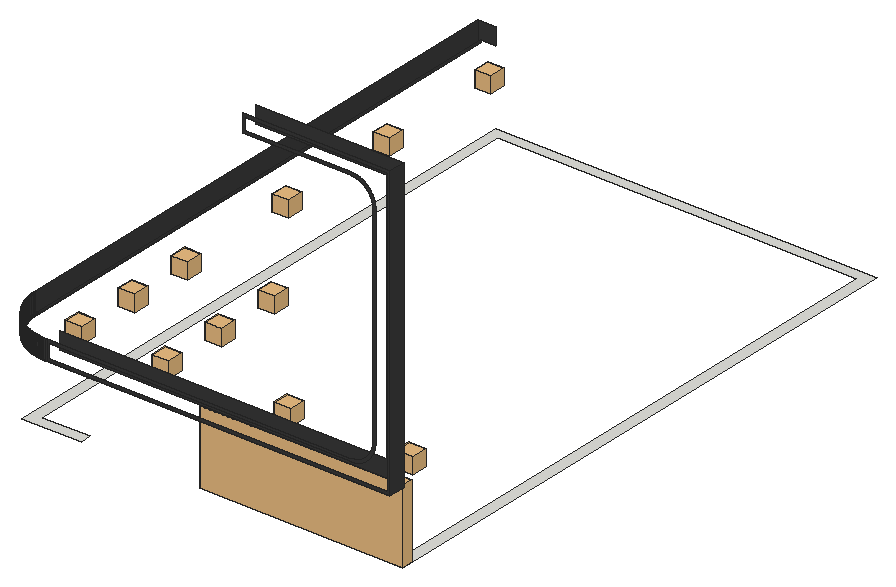
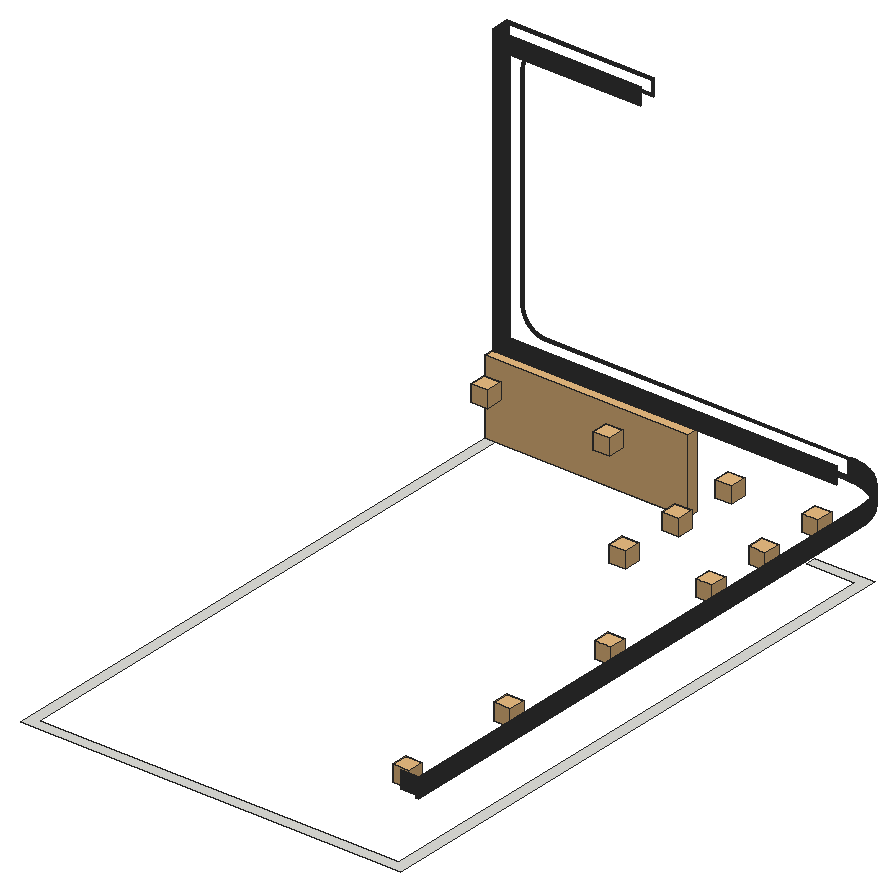
# SketchUp Ruby script. Lengths in inches.
U = 1.inch
M = Sketchup.active_model
def pt(a) = Geom::Point3d.new(a.map { |v| v * U })
def face(e, loops, mat)
  f = e.add_face(loops[0].map { |a| pt(a) })
  loops[1..].each { |l| e.add_face(l.map { |a| pt(a) }).erase! }
  f.material = f.back_material = mat if mat
  f
end
# faces: each face lists its corners as indices into pts; further lists are holes
def faces(e, pts, list, mat = nil) = list.each { |f| face(e, (f[0].is_a?(Array) ? f : [f]).map { |l| l.map { |i| pts[i] } }, mat) }
# xy, xz, yz: faces in a plane at the given z, y or x. An outline is a flat list of corners, or four numbers for a rectangle; further outlines are holes
def ring(l) = l.size == 4 ? [[l[0], l[1]], [l[2], l[1]], [l[2], l[3]], [l[0], l[3]]] : l.each_slice(2).to_a
def flat(e, list, mat, &to3) = list.each { |f| face(e, (f[0].is_a?(Array) ? f : [f]).map { |l| ring(l).map { |u, v| to3.(u, v) } }, mat) }
def xy(e, z, list, mat = nil) = flat(e, list, mat) { |x, y| [x, y, z] }
def xz(e, y, list, mat = nil) = flat(e, list, mat) { |x, z| [x, y, z] }
def yz(e, x, list, mat = nil) = flat(e, list, mat) { |y, z| [x, y, z] }
def lines(e, pts, list) = list.each { |a, b| e.add_line(pt(pts[a]), pt(pts[b])) }
# prism: a flat outline (further loops are holes) pulled along v
def prism(e, loops, v, mat = nil)
  f = face(e, loops, mat); d = Geom::Vector3d.new(v.map { |x| x * U })
  f.pushpull(f.normal.samedirection?(d) ? d.length : -d.length)
end
def box(e, o, s, mat = nil) = prism(e, [[o, [o[0] + s[0], o[1], o[2]], [o[0] + s[0], o[1] + s[1], o[2]], [o[0], o[1] + s[1], o[2]]]], [0, 0, s[2]], mat)
def at(x, y, z, deg = 0) = Geom::Transformation.translation(pt([x, y, z])) * Geom::Transformation.rotation(ORIGIN, Z_AXIS, deg.degrees)
def axes(o, x, y, z) = Geom::Transformation.new([*x, 0, *y, 0, *z, 0, *pt(o).to_a, 1])
def part(name) = M.definitions.add(name)
# library, detail: a bought-in or finely detailed component or shape, given as its bounding box
def library(name, o, s) = part(name).tap { |d| box(d.entities, o, s) }
def detail(e, o, s) = box(e.add_group.entities, o, s)
def put(e, d, t, mat = nil) = e.add_instance(d, t).tap { |i| i.material = mat if mat }
def group(e, t, mat = nil) = e.add_group.tap { |g| g.transformation = t; g.material = mat if mat }.entities
root = M.entities
M.materials.add("1496 AP 8293 CARBON COPY").color = [58, 58, 58]
c1 = library("Group\#5",[0,0,0],[165,9,60])
c2 = library("2",[-4.69,-4.69,-13.16],[13.38,13.38,13.16])
xy(root,69,[[14,84,62,84,62,93,23,93,23,555,314,555,314,93,158,93,158,84,323,84,323,564,14,564]])
xy(root,127,[[43.42,71,42.85,71.02,42.27,71.03,41.7,71.06,41.12,71.09,40.55,71.14,39.97,71.18,38.83,71.3,38.26,71.375,37.6875,71.46,37.12,71.54,35.98,71.74,35.42,71.85,34.85,71.96,34.29,72.08,33.73,72.22,33.17,72.35,32.61,72.5,32.06,72.65,31.5,72.8125,30.95,72.98,30.4,73.15,29.86,73.34,29.3125,73.52,28.77,73.72,28.23,73.92,27.7,74.13,27.16,74.35,26.63,74.57,26.1,74.8,25.58,75.04,24.54,75.54,24.02,75.8,23.51,76.0625,23.01,76.33,22.5,76.61,22,76.89,21.5,77.1875,21.01,77.48,20.52,77.79,20.04,78.1,19.55,78.42,19.08,78.74,18.14,79.4,17.67,79.74,17.21,80.09,15.86,81.17,15.42,81.54,14.56,82.3,14.13,82.69,13.71,83.08,13.3,83.48,12.48,84.3,12.08,84.71,11.69,85.13,11.3,85.56,10.54,86.42,10.17,86.86,9.09,88.21,8.74,88.67,8.4,89.14,7.74,90.08,7.42,90.55,7.1,91.04,6.79,91.52,6.48,92.01,6.1875,92.5,5.89,93,5.61,93.5,5.33,94.01,5.0625,94.51,4.8,95.02,4.54,95.54,4.04,96.58,3.8,97.1,3.57,97.63,3.35,98.16,3.13,98.7,2.92,99.23,2.72,99.77,2.52,100.3125,2.34,100.86,2.15,101.4,1.98,101.95,1.8125,102.5,1.65,103.06,1.5,103.61,1.35,104.17,1.22,104.73,1.08,105.29,0.96,105.85,0.85,106.42,0.74,106.98,0.54,108.12,0.46,108.6875,0.375,109.26,0.3,109.83,0.18,110.97,0.14,111.55,0.09,112.12,0.06,112.7,0.03,113.27,0.02,113.85,0,114.42,0,564,2,564,2,114.45,2.01,113.9,2.03,113.35,2.09,112.25,2.13,111.7,2.18,111.16,2.23,110.61,2.29,110.0625,2.36,109.52,2.43,108.97,2.7,107.35,2.92,106.27,3.04,105.73,3.16,105.2,3.29,104.66,3.43,104.13,3.73,103.07,3.89,102.55,4.06,102.02,4.23,101.5,4.41,100.98,4.6,100.46,4.79,99.95,4.99,99.4375,5.2,98.93,5.41,98.42,5.63,97.92,6.09,96.92,6.33,96.42,6.83,95.44,7.09,94.96,7.36,94.48,7.625,94,7.9,93.53,8.1875,93.06,8.48,92.59,8.78,92.125,9.08,91.67,9.39,91.21,9.7,90.76,10.02,90.3125,10.35,89.87,10.68,89.43,11.36,88.57,11.71,88.14,12.0625,87.72,12.42,87.31,13.16,86.49,13.53,86.09,13.92,85.69,14.3,85.3,14.69,84.92,15.09,84.53,15.49,84.16,16.31,83.42,16.72,83.0625,17.14,82.71,17.57,82.36,18.43,81.68,18.87,81.35,19.3125,81.02,19.76,80.7,20.21,80.39,20.67,80.08,21.125,79.78,21.59,79.48,22.06,79.1875,22.53,78.9,23,78.625,23.48,78.36,23.96,78.09,24.44,77.83,25.42,77.33,25.92,77.09,26.92,76.63,27.42,76.41,27.93,76.2,28.4375,75.99,28.95,75.79,29.46,75.6,29.98,75.41,30.5,75.23,31.02,75.06,31.55,74.89,32.07,74.73,33.13,74.43,33.66,74.29,34.2,74.16,34.73,74.04,35.27,73.92,36.35,73.7,37.97,73.43,38.52,73.36,39.0625,73.29,39.61,73.23,40.16,73.18,40.7,73.13,41.25,73.09,42.35,73.03,42.9,73.01,43.45,73,321,73,321,85,323,85,323,71]],"1496 AP 8293 CARBON COPY")
xz(root,71,[[43.42,127,44,143],[[44,127,323,127,323,363,203,363,203,349,291.24,349,291.47,348.99,291.71,348.99,291.94,348.98,292.18,348.96,292.41,348.94,292.65,348.92,292.88,348.9,293.12,348.875,293.35,348.85,293.58,348.8125,293.82,348.78,294.28,348.7,294.51,348.65,294.74,348.61,294.97,348.56,295.2,348.5,295.43,348.45,295.66,348.39,295.89,348.32,296.11,348.26,296.34,348.19,296.5625,348.12,296.79,348.04,297.01,347.97,297.23,347.89,297.45,347.8,297.67,347.72,298.11,347.54,298.32,347.44,298.54,347.35,298.75,347.25,298.96,347.14,299.17,347.04,299.59,346.82,299.8,346.7,300,346.59,300.4,346.35,300.61,346.22,300.8,346.1,301,345.97,301.2,345.83,301.39,345.7,301.58,345.5625,301.77,345.42,301.96,345.28,302.14,345.14,302.33,344.99,302.51,344.84,302.69,344.6875,302.87,344.53,303.04,344.375,303.22,344.22,303.39,344.06,303.56,343.89,303.73,343.73,303.89,343.56,304.06,343.39,304.22,343.22,304.375,343.04,304.53,342.87,304.6875,342.69,304.84,342.51,304.99,342.33,305.14,342.14,305.28,341.96,305.42,341.77,305.5625,341.58,305.7,341.39,305.83,341.2,305.97,341,306.1,340.8,306.22,340.61,306.35,340.4,306.59,340,306.7,339.8,306.82,339.59,307.04,339.17,307.14,338.96,307.25,338.75,307.35,338.54,307.44,338.32,307.54,338.11,307.72,337.67,307.8,337.45,307.89,337.23,307.97,337.01,308.04,336.79,308.12,336.5625,308.19,336.34,308.26,336.11,308.32,335.89,308.39,335.66,308.45,335.43,308.5,335.2,308.56,334.97,308.61,334.74,308.65,334.51,308.7,334.28,308.78,333.82,308.8125,333.58,308.85,333.35,308.875,333.12,308.9,332.88,308.92,332.65,308.94,332.41,308.96,332.18,308.98,331.94,308.99,331.71,308.99,331.47,309,331.24,309,160.76,308.99,160.53,308.99,160.29,308.98,160.06,308.96,159.82,308.94,159.59,308.92,159.35,308.9,159.12,308.875,158.88,308.85,158.65,308.8125,158.42,308.78,158.18,308.7,157.72,308.65,157.49,308.61,157.26,308.56,157.03,308.5,156.8,308.45,156.57,308.39,156.34,308.32,156.11,308.26,155.89,308.19,155.66,308.12,155.4375,308.04,155.21,307.97,154.99,307.89,154.77,307.8,154.55,307.72,154.33,307.54,153.89,307.44,153.68,307.35,153.46,307.25,153.25,307.14,153.04,307.04,152.83,306.82,152.41,306.7,152.2,306.59,152,306.35,151.6,306.22,151.39,306.1,151.2,305.97,151,305.83,150.8,305.7,150.61,305.5625,150.42,305.42,150.23,305.28,150.04,305.14,149.86,304.99,149.67,304.84,149.49,304.6875,149.31,304.53,149.13,304.375,148.96,304.22,148.78,304.06,148.61,303.89,148.44,303.73,148.27,303.56,148.11,303.39,147.94,303.22,147.78,303.04,147.625,302.87,147.47,302.69,147.3125,302.51,147.16,302.33,147.01,302.14,146.86,301.96,146.72,301.77,146.58,301.58,146.4375,301.39,146.3,301.2,146.17,301,146.03,300.8,145.9,300.61,145.78,300.4,145.65,300,145.41,299.8,145.3,299.59,145.18,299.17,144.96,298.96,144.86,298.75,144.75,298.54,144.65,298.32,144.56,298.11,144.46,297.67,144.28,297.45,144.2,297.23,144.11,297.01,144.03,296.79,143.96,296.5625,143.88,296.34,143.81,296.11,143.74,295.89,143.68,295.66,143.61,295.43,143.55,295.2,143.5,294.97,143.44,294.74,143.39,294.51,143.35,294.28,143.3,293.82,143.22,293.58,143.1875,293.35,143.15,293.12,143.125,292.88,143.1,292.65,143.08,292.41,143.06,292.18,143.04,291.94,143.02,291.71,143.01,291.47,143.01,291.24,143,44,143],[46,129,46,141,291.26,141,291.52,141.01,291.79,141.02,292.31,141.04,292.57,141.0625,292.83,141.08,293.61,141.17,294.39,141.29,294.64,141.33,294.9,141.38,295.16,141.4375,295.41,141.49,295.67,141.55,295.92,141.62,296.18,141.68,296.68,141.82,297.18,141.98,297.43,142.0625,297.68,142.15,297.92,142.24,298.17,142.33,298.41,142.42,298.65,142.52,299.13,142.73,299.375,142.84,299.61,142.95,299.85,143.0625,300.08,143.18,300.3125,143.3,300.54,143.42,301,143.68,301.23,143.8125,301.45,143.95,302.11,144.37,302.33,144.52,302.54,144.67,302.76,144.82,302.97,144.97,303.18,145.13,303.38,145.29,303.59,145.46,303.99,145.79,304.1875,145.96,304.38,146.14,304.58,146.3125,304.77,146.49,304.96,146.67,305.14,146.86,305.33,147.04,305.51,147.23,305.6875,147.42,305.86,147.62,306.04,147.8125,306.21,148.01,306.54,148.41,306.71,148.62,306.87,148.82,307.03,149.03,307.18,149.24,307.33,149.46,307.48,149.67,307.63,149.89,308.05,150.55,308.1875,150.77,308.32,151,308.58,151.46,308.7,151.6875,308.82,151.92,308.9375,152.15,309.05,152.39,309.16,152.625,309.27,152.87,309.48,153.35,309.58,153.59,309.67,153.83,309.76,154.08,309.85,154.32,309.9375,154.57,310.02,154.82,310.18,155.32,310.32,155.82,310.38,156.08,310.45,156.33,310.51,156.59,310.5625,156.84,310.62,157.1,310.67,157.36,310.71,157.61,310.83,158.39,310.92,159.17,310.9375,159.43,310.96,159.69,310.98,160.21,310.99,160.48,311,160.74,311,331.26,310.99,331.52,310.98,331.79,310.96,332.31,310.9375,332.57,310.92,332.83,310.83,333.61,310.71,334.39,310.67,334.64,310.62,334.9,310.5625,335.16,310.51,335.41,310.45,335.67,310.38,335.92,310.32,336.18,310.18,336.68,310.02,337.18,309.9375,337.43,309.85,337.68,309.76,337.92,309.67,338.17,309.58,338.41,309.48,338.65,309.27,339.13,309.16,339.375,309.05,339.61,308.9375,339.85,308.82,340.08,308.7,340.3125,308.58,340.54,308.32,341,308.1875,341.23,308.05,341.45,307.63,342.11,307.48,342.33,307.33,342.54,307.18,342.76,307.03,342.97,306.87,343.18,306.71,343.38,306.54,343.59,306.21,343.99,306.04,344.1875,305.86,344.38,305.6875,344.58,305.51,344.77,305.33,344.96,305.14,345.14,304.96,345.33,304.77,345.51,304.58,345.6875,304.38,345.86,304.1875,346.04,303.99,346.21,303.59,346.54,303.38,346.71,303.18,346.87,302.97,347.03,302.76,347.18,302.54,347.33,302.33,347.48,302.11,347.63,301.45,348.05,301.23,348.1875,301,348.32,300.54,348.58,300.3125,348.7,300.08,348.82,299.85,348.9375,299.61,349.05,299.375,349.16,299.13,349.27,298.65,349.48,298.41,349.58,298.17,349.67,297.92,349.76,297.68,349.85,297.43,349.9375,297.18,350.02,296.68,350.18,296.18,350.32,295.92,350.38,295.67,350.45,295.41,350.51,295.16,350.5625,294.9,350.62,294.64,350.67,294.39,350.71,293.61,350.83,292.83,350.92,292.57,350.9375,292.31,350.96,291.79,350.98,291.52,350.99,291.26,351,205,351,205,361,321,361,321,129]]],"1496 AP 8293 CARBON COPY")
xz(root,73,[[43.45,127,44,129]],"1496 AP 8293 CARBON COPY")
xz(root,85,[[321,127,321,129,44,129,44,143,309,143,309,349,203,349,203,363,323,363,323,127]],"1496 AP 8293 CARBON COPY")
xz(root,564,[[0,127,0,143,14,143,14,129,2,129,2,127]],"1496 AP 8293 CARBON COPY")
yz(root,0,[[114.42,127,115,143],[115,127,564,143]],"1496 AP 8293 CARBON COPY")
yz(root,2,[[114.45,127,115,129],[115,127,564,129]],"1496 AP 8293 CARBON COPY")
yz(root,321,[[73,127,85,129]],"1496 AP 8293 CARBON COPY")
yz(root,323,[[71,127,85,363]],"1496 AP 8293 CARBON COPY")
p = [[41.7,71.06,143],[41.7,71.06,127],[42.27,71.03,127],[42.27,71.03,143],[42.85,71.02,127],[42.85,71.02,143],
  [43.42,71,127],[43.42,71,143],[39.97,71.18,143],[39.97,71.18,127],[40.55,71.14,127],[40.55,71.14,143],
  [41.12,71.09,127],[41.12,71.09,143],[38.83,71.3,143],[38.83,71.3,127],[39.4,71.24,127],[39.4,71.24,143],
  [38.26,71.375,143],[38.26,71.375,127],[37.6875,71.46,143],[37.6875,71.46,127],[36.55,71.64,143],[36.55,71.64,127],
  [37.12,71.54,127],[37.12,71.54,143],[35.98,71.74,143],[35.98,71.74,127],[35.42,71.85,143],[35.42,71.85,127],
  [34.85,71.96,143],[34.85,71.96,127],[34.29,72.08,143],[34.29,72.08,127],[33.73,72.22,143],[33.73,72.22,127],
  [33.17,72.35,143],[33.17,72.35,127],[32.61,72.5,143],[32.61,72.5,127],[32.06,72.65,143],[32.06,72.65,127],
  [31.5,72.8125,143],[31.5,72.8125,127],[30.95,72.98,143],[30.95,72.98,127],[30.4,73.15,143],[30.4,73.15,127],
  [41.8,73.06,129],[42.35,73.03,129],[42.35,73.03,127],[41.8,73.06,127],[42.9,73.01,129],[42.9,73.01,127],
  [43.45,73,129],[43.45,73,127],[40.16,73.18,129],[40.7,73.13,129],[40.7,73.13,127],[40.16,73.18,127],
  [41.25,73.09,129],[41.25,73.09,127],[29.86,73.34,143],[29.86,73.34,127],[39.0625,73.29,129],[39.61,73.23,129],
  [39.61,73.23,127],[39.0625,73.29,127],[29.3125,73.52,143],[29.3125,73.52,127],[38.52,73.36,129],[38.52,73.36,127],
  [37.43,73.52,129],[37.97,73.43,129],[37.97,73.43,127],[37.43,73.52,127],[28.77,73.72,143],[28.77,73.72,127],
  [36.89,73.61,129],[36.89,73.61,127],[36.35,73.7,129],[36.35,73.7,127],[28.23,73.92,143],[28.23,73.92,127],
  [35.81,73.81,129],[35.81,73.81,127],[35.27,73.92,129],[35.27,73.92,127],[27.7,74.13,143],[27.7,74.13,127],
  [34.73,74.04,129],[34.73,74.04,127],[34.2,74.16,129],[34.2,74.16,127],[27.16,74.35,143],[27.16,74.35,127],
  [33.66,74.29,129],[33.66,74.29,127],[26.63,74.57,143],[26.63,74.57,127],[33.13,74.43,129],[33.13,74.43,127],
  [32.6,74.58,129],[32.6,74.58,127],[26.1,74.8,143],[26.1,74.8,127],[32.07,74.73,129],[32.07,74.73,127],
  [31.55,74.89,129],[31.55,74.89,127],[25.58,75.04,143],[25.58,75.04,127],[31.02,75.06,129],[31.02,75.06,127],
  [25.06,75.29,143],[25.06,75.29,127],[30.5,75.23,129],[30.5,75.23,127],[29.98,75.41,129],[29.98,75.41,127],
  [24.54,75.54,143],[24.54,75.54,127],[29.46,75.6,129],[29.46,75.6,127],[24.02,75.8,143],[24.02,75.8,127],
  [28.95,75.79,129],[28.95,75.79,127],[23.51,76.0625,143],[23.51,76.0625,127],[28.4375,75.99,129],[28.4375,75.99,127],
  [27.93,76.2,129],[27.93,76.2,127],[23.01,76.33,143],[23.01,76.33,127],[27.42,76.41,129],[27.42,76.41,127],
  [22.5,76.61,143],[22.5,76.61,127],[26.92,76.63,129],[26.92,76.63,127],[22,76.89,143],[22,76.89,127],
  [26.42,76.86,129],[26.42,76.86,127],[21.5,77.1875,143],[21.5,77.1875,127],[25.92,77.09,129],[25.92,77.09,127],
  [25.42,77.33,129],[25.42,77.33,127],[21.01,77.48,143],[21.01,77.48,127],[24.93,77.58,129],[24.93,77.58,127],
  [20.52,77.79,143],[20.52,77.79,127],[24.44,77.83,129],[24.44,77.83,127],[20.04,78.1,143],[20.04,78.1,127],
  [23.96,78.09,129],[23.96,78.09,127],[19.55,78.42,143],[19.55,78.42,127],[23.48,78.36,129],[23.48,78.36,127],
  [19.08,78.74,143],[19.08,78.74,127],[23,78.625,129],[23,78.625,127],[22.53,78.9,129],[22.53,78.9,127],
  [18.61,79.07,143],[18.61,79.07,127],[22.06,79.1875,129],[22.06,79.1875,127],[18.14,79.4,143],[18.14,79.4,127],
  [21.59,79.48,129],[21.59,79.48,127],[17.67,79.74,143],[17.67,79.74,127],[21.125,79.78,129],[21.125,79.78,127],
  [17.21,80.09,143],[17.21,80.09,127],[20.67,80.08,129],[20.67,80.08,127],[16.76,80.45,143],[16.76,80.45,127],
  [20.21,80.39,129],[20.21,80.39,127],[16.31,80.81,143],[16.31,80.81,127],[19.76,80.7,129],[19.76,80.7,127],
  [19.3125,81.02,129],[19.3125,81.02,127],[15.86,81.17,143],[15.86,81.17,127],[18.87,81.35,129],[18.87,81.35,127],
  [15.42,81.54,143],[15.42,81.54,127],[18.43,81.68,129],[18.43,81.68,127],[14.99,81.92,143],[14.99,81.92,127],
  [18,82.02,129],[18,82.02,127],[14.56,82.3,143],[14.56,82.3,127],[17.57,82.36,129],[17.57,82.36,127],
  [14.13,82.69,143],[14.13,82.69,127],[17.14,82.71,129],[17.14,82.71,127],[13.71,83.08,143],[13.71,83.08,127],
  [16.72,83.0625,129],[16.72,83.0625,127],[13.3,83.48,143],[13.3,83.48,127],[16.31,83.42,129],[16.31,83.42,127],
  [15.9,83.79,129],[15.9,83.79,127],[12.89,83.89,143],[12.89,83.89,127],[15.49,84.16,129],[15.49,84.16,127],
  [12.48,84.3,143],[12.48,84.3,127],[15.09,84.53,129],[15.09,84.53,127],[12.08,84.71,143],[12.08,84.71,127],
  [14.69,84.92,129],[14.69,84.92,127],[11.69,85.13,143],[11.69,85.13,127],[14.3,85.3,129],[14.3,85.3,127],
  [11.3,85.56,143],[11.3,85.56,127],[13.92,85.69,129],[13.92,85.69,127],[10.92,85.99,143],[10.92,85.99,127],
  [13.53,86.09,129],[13.53,86.09,127],[10.54,86.42,143],[10.54,86.42,127],[13.16,86.49,129],[13.16,86.49,127],
  [10.17,86.86,143],[10.17,86.86,127],[12.79,86.9,129],[12.79,86.9,127],[9.81,87.31,143],[9.81,87.31,127],
  [12.42,87.31,129],[12.42,87.31,127],[9.45,87.76,143],[9.45,87.76,127],[12.0625,87.72,129],[12.0625,87.72,127],
  [11.71,88.14,129],[11.71,88.14,127],[9.09,88.21,143],[9.09,88.21,127],[11.36,88.57,129],[11.36,88.57,127],
  [8.74,88.67,143],[8.74,88.67,127],[11.02,89,129],[11.02,89,127],[8.4,89.14,143],[8.4,89.14,127],
  [10.68,89.43,129],[10.68,89.43,127],[8.07,89.61,143],[8.07,89.61,127],[10.35,89.87,129],[10.35,89.87,127],
  [7.74,90.08,143],[7.74,90.08,127],[10.02,90.3125,129],[10.02,90.3125,127],[7.42,90.55,143],[7.42,90.55,127],
  [9.7,90.76,129],[9.7,90.76,127],[7.1,91.04,143],[7.1,91.04,127],[9.39,91.21,129],[9.39,91.21,127],
  [6.79,91.52,143],[6.79,91.52,127],[9.08,91.67,129],[9.08,91.67,127],[6.48,92.01,143],[6.48,92.01,127],
  [8.78,92.125,129],[8.78,92.125,127],[6.1875,92.5,143],[6.1875,92.5,127],[8.48,92.59,129],[8.48,92.59,127],
  [5.89,93,143],[5.89,93,127],[8.1875,93.06,129],[8.1875,93.06,127],[5.61,93.5,143],[5.61,93.5,127],
  [7.9,93.53,129],[7.9,93.53,127],[5.33,94.01,143],[5.33,94.01,127],[7.625,94,129],[7.625,94,127],
  [5.0625,94.51,143],[5.0625,94.51,127],[7.36,94.48,129],[7.36,94.48,127],[4.8,95.02,143],[4.8,95.02,127],
  [7.09,94.96,129],[7.09,94.96,127],[4.54,95.54,143],[4.54,95.54,127],[6.83,95.44,129],[6.83,95.44,127],
  [6.58,95.93,129],[6.58,95.93,127],[4.29,96.06,143],[4.29,96.06,127],[6.33,96.42,129],[6.33,96.42,127],
  [4.04,96.58,143],[4.04,96.58,127],[6.09,96.92,129],[6.09,96.92,127],[3.8,97.1,143],[3.8,97.1,127],
  [5.86,97.42,129],[5.86,97.42,127],[3.57,97.63,143],[3.57,97.63,127],[5.63,97.92,129],[5.63,97.92,127],
  [3.35,98.16,143],[3.35,98.16,127],[5.41,98.42,129],[5.41,98.42,127],[3.13,98.7,143],[3.13,98.7,127],
  [5.2,98.93,129],[5.2,98.93,127],[2.92,99.23,143],[2.92,99.23,127],[4.99,99.4375,129],[4.99,99.4375,127],
  [2.72,99.77,143],[2.72,99.77,127],[4.79,99.95,129],[4.79,99.95,127],[2.52,100.3125,143],[2.52,100.3125,127],
  [4.6,100.46,129],[4.6,100.46,127],[2.34,100.86,143],[2.34,100.86,127],[4.41,100.98,129],[4.41,100.98,127],
  [2.15,101.4,143],[2.15,101.4,127],[4.23,101.5,129],[4.23,101.5,127],[1.98,101.95,143],[1.98,101.95,127],
  [4.06,102.02,129],[4.06,102.02,127],[1.8125,102.5,143],[1.8125,102.5,127],[3.89,102.55,129],[3.89,102.55,127],
  [1.65,103.06,143],[1.65,103.06,127],[3.73,103.07,129],[3.73,103.07,127],[1.5,103.61,143],[1.5,103.61,127],
  [3.58,103.6,129],[3.58,103.6,127],[1.35,104.17,143],[1.35,104.17,127],[3.43,104.13,129],[3.43,104.13,127],
  [3.29,104.66,129],[3.29,104.66,127],[1.22,104.73,143],[1.22,104.73,127],[1.08,105.29,143],[1.08,105.29,127],
  [3.16,105.2,129],[3.16,105.2,127],[3.04,105.73,129],[3.04,105.73,127],[0.96,105.85,143],[0.96,105.85,127],
  [2.92,106.27,129],[2.92,106.27,127],[0.85,106.42,143],[0.85,106.42,127],[2.81,106.81,129],[2.81,106.81,127],
  [0.74,106.98,143],[0.74,106.98,127],[2.7,107.35,129],[2.7,107.35,127],[0.64,107.55,143],[0.64,107.55,127],
  [2.61,107.89,129],[2.61,107.89,127],[0.54,108.12,143],[0.54,108.12,127],[2.52,108.43,129],[2.52,108.43,127],
  [0.46,108.6875,143],[0.46,108.6875,127],[2.43,108.97,129],[2.43,108.97,127],[0.375,109.26,143],[0.375,109.26,127],
  [2.36,109.52,129],[2.36,109.52,127],[0.3,109.83,143],[0.3,109.83,127],[2.29,110.0625,129],[2.29,110.0625,127],
  [0.24,110.4,143],[0.24,110.4,127],[2.23,110.61,129],[2.23,110.61,127],[0.18,110.97,143],[0.18,110.97,127],
  [2.18,111.16,129],[2.18,111.16,127],[0.14,111.55,143],[0.14,111.55,127],[2.13,111.7,129],[2.13,111.7,127],
  [0.09,112.12,143],[0.09,112.12,127],[2.09,112.25,129],[2.09,112.25,127],[0.06,112.7,143],[0.06,112.7,127],
  [2.06,112.8,129],[2.06,112.8,127],[0.03,113.27,143],[0.03,113.27,127],[2.03,113.35,129],[2.03,113.35,127],
  [0.02,113.85,143],[0.02,113.85,127],[2.01,113.9,129],[2.01,113.9,127],[0,114.42,143],[0,114.42,127],
  [2,114.45,129],[2,114.45,127]]
faces(root,p,[[0,1,2,3],[3,2,4,5],[5,4,6,7],[8,9,10,11],[11,10,12,13],[13,12,1,0],[14,15,16,17],[17,16,9,8],
  [18,19,15,14],[20,21,19,18],[22,23,24,25],[25,24,21,20],[26,27,23,22],[28,29,27,26],[30,31,29,28],[32,33,31,30],
  [34,35,33,32],[36,37,35,34],[38,39,37,36],[40,41,39,38],[42,43,41,40],[44,45,43,42],[46,47,45,44],[48,49,50,51],
  [49,52,53,50],[52,54,55,53],[56,57,58,59],[57,60,61,58],[60,48,51,61],[62,63,47,46],[64,65,66,67],[65,56,59,66],
  [68,69,63,62],[70,64,67,71],[72,73,74,75],[73,70,71,74],[76,77,69,68],[78,72,75,79],[80,78,79,81],[82,83,77,76],
  [84,80,81,85],[86,84,85,87],[88,89,83,82],[90,86,87,91],[92,90,91,93],[94,95,89,88],[96,92,93,97],[98,99,95,94],
  [100,96,97,101],[102,100,101,103],[104,105,99,98],[106,102,103,107],[108,106,107,109],[110,111,105,104],[112,108,109,113],[114,115,111,110],
  [116,112,113,117],[118,116,117,119],[120,121,115,114],[122,118,119,123],[124,125,121,120],[126,122,123,127],[128,129,125,124],[130,126,127,131],
  [132,130,131,133],[134,135,129,128],[136,132,133,137],[138,139,135,134],[140,136,137,141],[142,143,139,138],[144,140,141,145],[146,147,143,142],
  [148,144,145,149],[150,148,149,151],[152,153,147,146],[154,150,151,155],[156,157,153,152],[158,154,155,159],[160,161,157,156],[162,158,159,163],
  [164,165,161,160],[166,162,163,167],[168,169,165,164],[170,166,167,171],[172,170,171,173],[174,175,169,168],[176,172,173,177],[178,179,175,174],
  [180,176,177,181],[182,183,179,178],[184,180,181,185],[186,187,183,182],[188,184,185,189],[190,191,187,186],[192,188,189,193],[194,195,191,190],
  [196,192,193,197],[198,196,197,199],[200,201,195,194],[202,198,199,203],[204,205,201,200],[206,202,203,207],[208,209,205,204],[210,206,207,211],
  [212,213,209,208],[214,210,211,215],[216,217,213,212],[218,214,215,219],[220,221,217,216],[222,218,219,223],[224,225,221,220],[226,222,223,227],
  [228,226,227,229],[230,231,225,224],[232,228,229,233],[234,235,231,230],[236,232,233,237],[238,239,235,234],[240,236,237,241],[242,243,239,238],
  [244,240,241,245],[246,247,243,242],[248,244,245,249],[250,251,247,246],[252,248,249,253],[254,255,251,250],[256,252,253,257],[258,259,255,254],
  [260,256,257,261],[262,263,259,258],[264,260,261,265],[266,267,263,262],[268,264,265,269],[270,268,269,271],[272,273,267,266],[274,270,271,275],
  [276,277,273,272],[278,274,275,279],[280,281,277,276],[282,278,279,283],[284,285,281,280],[286,282,283,287],[288,289,285,284],[290,286,287,291],
  [292,293,289,288],[294,290,291,295],[296,297,293,292],[298,294,295,299],[300,301,297,296],[302,298,299,303],[304,305,301,300],[306,302,303,307],
  [308,309,305,304],[310,306,307,311],[312,313,309,308],[314,310,311,315],[316,317,313,312],[318,314,315,319],[320,321,317,316],[322,318,319,323],
  [324,325,321,320],[326,322,323,327],[328,329,325,324],[330,326,327,331],[332,333,329,328],[334,330,331,335],[336,334,335,337],[338,339,333,332],
  [340,336,337,341],[342,343,339,338],[344,340,341,345],[346,347,343,342],[348,344,345,349],[350,351,347,346],[352,348,349,353],[354,355,351,350],
  [356,352,353,357],[358,359,355,354],[360,356,357,361],[362,363,359,358],[364,360,361,365],[366,367,363,362],[368,364,365,369],[370,371,367,366],
  [372,368,369,373],[374,375,371,370],[376,372,373,377],[378,379,375,374],[380,376,377,381],[382,383,379,378],[384,380,381,385],[386,387,383,382],
  [388,384,385,389],[390,391,387,386],[392,388,389,393],[394,395,391,390],[396,392,393,397],[398,399,395,394],[400,396,397,401],[402,400,401,403],
  [404,405,399,398],[406,407,405,404],[408,402,403,409],[410,408,409,411],[412,413,407,406],[414,410,411,415],[416,417,413,412],[418,414,415,419],
  [420,421,417,416],[422,418,419,423],[424,425,421,420],[426,422,423,427],[428,429,425,424],[430,426,427,431],[432,433,429,428],[434,430,431,435],
  [436,437,433,432],[438,434,435,439],[440,441,437,436],[442,438,439,443],[444,445,441,440],[446,442,443,447],[448,449,445,444],[450,446,447,451],
  [452,453,449,448],[454,450,451,455],[456,457,453,452],[458,454,455,459],[460,461,457,456],[462,458,459,463],[464,465,461,460],[466,462,463,467],
  [468,469,465,464],[470,466,467,471],[472,473,469,468],[474,470,471,475]],"1496 AP 8293 CARBON COPY")
put(root,c1,at(158,84,69))
put(root,c2,at(28.5,227.5,130.01))
put(root,c2,at(28.5,173.75,130.01))
put(root,c2,at(28.5,120,130.01))
put(root,c2,at(28.5,330,130.01))
put(root,c2,at(28.5,432.5,130.01))
put(root,c2,at(28.5,535,130.01))
put(root,c2,at(99,227.5,130.01))
put(root,c2,at(99,120,130.01))
put(root,c2,at(99,173.75,130.01))
put(root,c2,at(198,120,130.01))
put(root,c2,at(297,120,130.01))
